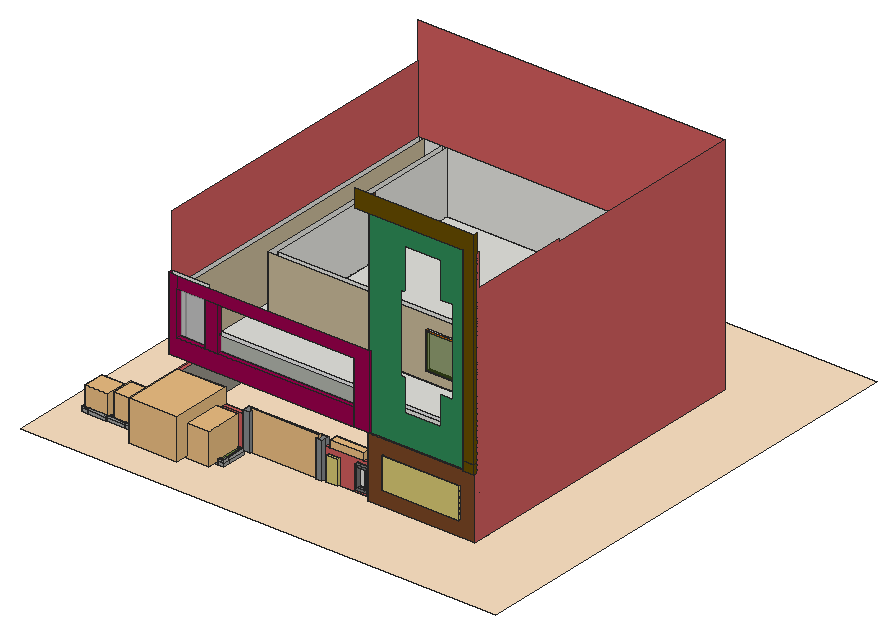
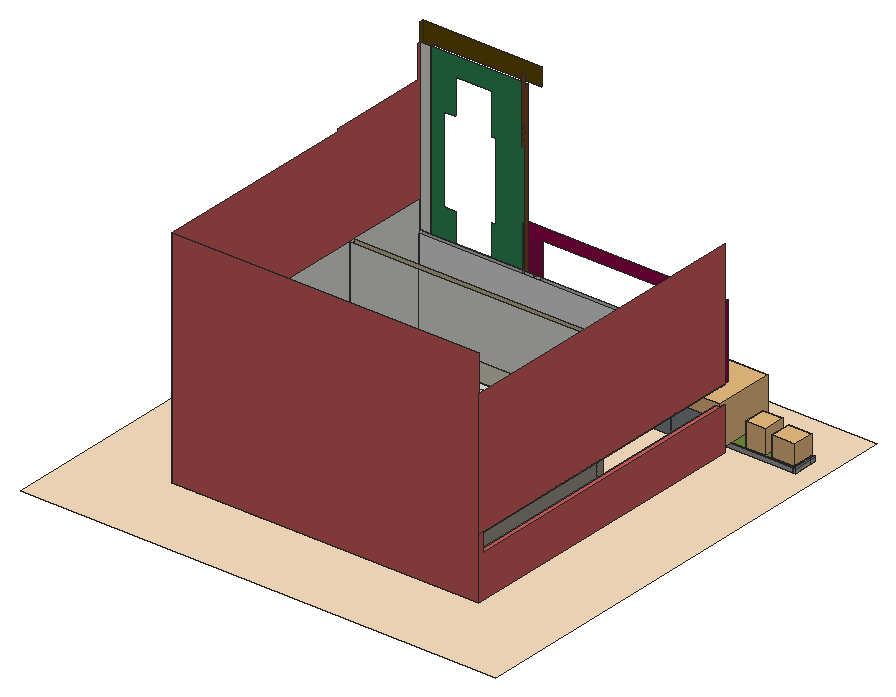
# SketchUp Ruby script. Lengths in inches.
U = 1.inch
M = Sketchup.active_model
def pt(a) = Geom::Point3d.new(a.map { |v| v * U })
def face(e, loops, mat)
  f = e.add_face(loops[0].map { |a| pt(a) })
  loops[1..].each { |l| e.add_face(l.map { |a| pt(a) }).erase! }
  f.material = f.back_material = mat if mat
  f
end
# faces: each face lists its corners as indices into pts; further lists are holes
def faces(e, pts, list, mat = nil) = list.each { |f| face(e, (f[0].is_a?(Array) ? f : [f]).map { |l| l.map { |i| pts[i] } }, mat) }
# xy, xz, yz: faces in a plane at the given z, y or x. An outline is a flat list of corners, or four numbers for a rectangle; further outlines are holes
def ring(l) = l.size == 4 ? [[l[0], l[1]], [l[2], l[1]], [l[2], l[3]], [l[0], l[3]]] : l.each_slice(2).to_a
def flat(e, list, mat, &to3) = list.each { |f| face(e, (f[0].is_a?(Array) ? f : [f]).map { |l| ring(l).map { |u, v| to3.(u, v) } }, mat) }
def xy(e, z, list, mat = nil) = flat(e, list, mat) { |x, y| [x, y, z] }
def xz(e, y, list, mat = nil) = flat(e, list, mat) { |x, z| [x, y, z] }
def yz(e, x, list, mat = nil) = flat(e, list, mat) { |y, z| [x, y, z] }
def lines(e, pts, list) = list.each { |a, b| e.add_line(pt(pts[a]), pt(pts[b])) }
# prism: a flat outline (further loops are holes) pulled along v
def prism(e, loops, v, mat = nil)
  f = face(e, loops, mat); d = Geom::Vector3d.new(v.map { |x| x * U })
  f.pushpull(f.normal.samedirection?(d) ? d.length : -d.length)
end
def box(e, o, s, mat = nil) = prism(e, [[o, [o[0] + s[0], o[1], o[2]], [o[0] + s[0], o[1] + s[1], o[2]], [o[0], o[1] + s[1], o[2]]]], [0, 0, s[2]], mat)
def at(x, y, z, deg = 0) = Geom::Transformation.translation(pt([x, y, z])) * Geom::Transformation.rotation(ORIGIN, Z_AXIS, deg.degrees)
def axes(o, x, y, z) = Geom::Transformation.new([*x, 0, *y, 0, *z, 0, *pt(o).to_a, 1])
def part(name) = M.definitions.add(name)
# library, detail: a bought-in or finely detailed component or shape, given as its bounding box
def library(name, o, s) = part(name).tap { |d| box(d.entities, o, s) }
def detail(e, o, s) = box(e.add_group.entities, o, s)
def put(e, d, t, mat = nil) = e.add_instance(d, t).tap { |i| i.material = mat if mat }
def group(e, t, mat = nil) = e.add_group.tap { |g| g.transformation = t; g.material = mat if mat }.entities
root = M.entities
M.materials.add("PDM_Concrete_02N").color = [160, 160, 159]
M.materials.add("PDM_Concrete_02N-1").color = [160, 160, 159]
M.materials.add("PDM_Grass_03").color = [113, 137, 58]
M.materials.add("[0012_Bisque]").color = [255, 228, 196]
M.materials.add("[0017_IndianRed]").color = [205, 92, 92]
M.materials.add("[0074_SeaGreen]").color = [46, 139, 87]
M.materials.add("[Blacktop Old 01]").color = [132, 136, 139]
M.materials.add("[Color A03]").color = [255, 101, 101]
M.materials.add("[Color C06]").color = [204, 102, 0]
M.materials.add("[Color D08]").color = [102, 76, 0]
M.materials.add("[Color L11]").color = [153, 0, 76]
M.materials.add("[Color M05]").color = [114, 114, 114]
M.materials.add("[Formica Graystone]").color = [149, 146, 135]
M.materials.add("[Mirror 02]").color = [229, 229, 229]
M.materials.add("[Quartz Light Brown]").color = [199, 184, 152]
M.materials.add("[Translucent Glass Blue]").color = [100, 149, 237]
M.materials["[Translucent Glass Blue]"].alpha = 0.5
M.materials.add("[Translucent Glass Dark Green]").color = [62, 91, 5]
M.materials["[Translucent Glass Dark Green]"].alpha = 0.5
M.materials.add("[Translucent Resin Crush Gray]").color = [184, 184, 184]
M.materials["[Translucent Resin Crush Gray]"].alpha = 0.8
M.materials.add("[Wood Board Cork]").color = [215, 201, 115]
M.materials.add("[Wood Floor Parquet]").color = [145, 89, 39]
M.materials.add("[Wood Veneer 01]").color = [120, 70, 37]
c1 = library("gate",[-17.08,19.83,-10.33],[162.44,1,145.04])
c2 = part("255x125 HB kerb.skp\#1")
prism(c2.entities,[[[35.98,4.92,10.04],[35.98,1.15,10.04],[35.98,0.9375,9.96],[35.98,0.8125,9.77],[35.98,0,6.1],[35.98,0,0],[35.98,4.92,0]]],[-35.98,0,0])
c3 = part("305x125 HB external kerb.skp")
xy(c3.entities,0,[[0,0,0,4.92,7.09,4.92,7.09,12.01,12.01,12.01,12.01,0]])
xy(c3.entities,10.04,[[0,1.15,10.86,1.15,10.86,12.01,7.09,12.01,7.09,4.92,0,4.92]])
xz(c3.entities,0,[[0,0,12.01,6.1]])
xz(c3.entities,4.92,[[0,0,7.09,10.04]])
xz(c3.entities,12.01,[[7.09,0,7.09,10.04,10.86,10.04,11.07,9.96,11.19,9.77,12.01,6.1,12.01,0]])
yz(c3.entities,0,[[0,0,0,6.1,0.8125,9.77,0.9375,9.96,1.15,10.04,4.92,10.04,4.92,0]])
yz(c3.entities,7.09,[[4.92,0,12.01,10.04]])
yz(c3.entities,12.01,[[0,0,12.01,6.1]])
p = [[0,0.8125,9.77],[0,0,6.1],[12.01,0,6.1],[11.19,0.8125,9.77],[12.01,12.01,6.1],[11.19,12.01,9.77],
  [0,0.9375,9.96],[11.07,0.9375,9.96],[11.07,12.01,9.96],[0,1.15,10.04],[10.86,1.15,10.04],[10.86,12.01,10.04]]
faces(c3.entities,p,[[0,1,2,3],[3,2,4,5],[6,0,3,7],[7,3,5,8],[9,6,7,10],[10,7,8,11]])
c4 = library("Vase_plant.skp",[-29.68,-24.2,-1.65],[45.82,40.28,40.94])
c5 = library("Aralia.skp\#1",[-13.5,-14.26,0],[27.8,28.98,28.64])
c6 = library("bamboo2.skp\#1",[-10.58,-11.09,0],[94.17,118.22,79.29])
c7 = library("Monstera.skp\#1",[-40.08,-33.23,-2.65],[72.39,71.54,61.35])
c8 = part("flowers")
xy(c8.entities,8.27,[[6.7,5.98,275.44,49.6875]],"PDM_Grass_03")
xz(c8.entities,5.98,[[6.7,0,275.44,8.27]])
xz(c8.entities,49.6875,[[6.7,0,6.9375,8.27],[6.9375,0,275.44,8.27],[6.9375,8.27,275.44,10.04]],"PDM_Concrete_02N")
yz(c8.entities,6.7,[[5.98,0,49.6875,8.27]])
yz(c8.entities,275.44,[[5.98,0,49.6875,8.27]])
p = [[2.02,1.3,0],[2.02,40.67,0]]
lines(c8.entities,p,[[0,1]])
put(c8.entities,c2,at(14.42,1.3,0),"PDM_Concrete_02N-1")
put(c8.entities,c3,at(268.36,1.3,0),"PDM_Concrete_02N-1")
put(c8.entities,c3,at(2.02,13.31,0,-90),"PDM_Concrete_02N-1")
put(c8.entities,c2,at(50.8,1.3,0),"PDM_Concrete_02N-1")
put(c8.entities,c2,at(87.18,1.3,0),"PDM_Concrete_02N-1")
put(c8.entities,c2,at(123.55,1.3,0),"PDM_Concrete_02N-1")
put(c8.entities,c2,at(159.77,1.3,0),"PDM_Concrete_02N-1")
put(c8.entities,c2,at(195.99,1.3,0),"PDM_Concrete_02N-1")
put(c8.entities,c2,at(232.21,1.3,0),"PDM_Concrete_02N-1")
put(c8.entities,c2,at(280.36,13.7,0,90),"PDM_Concrete_02N-1")
put(c8.entities,c2,at(2.02,49.6875,0,-90),"PDM_Concrete_02N-1")
put(c8.entities,c4,at(36.73,27.57,8.27))
put(c8.entities,c5,axes([82.45,23.77,8.27],[1.4,0,0],[0,1.43,0],[0,0,1.63]))
put(c8.entities,c6,at(140.88,-31.91,8.22))
put(c8.entities,c7,at(227.05,18.7,8.27,-180))
c9 = library("APU-ABUS-AZ18C-4-510B-36-CU",[3.59,-10.3125,0.03],[37.07,9.01,7.97])
xy(root,0,[[554.6,156.04,755.73,165.04],[755.73,156.04,765.04,165.04],[308.48,159.04,322.39,165.04],[450.54,159.04,462.67,165.04],[165.04,165.04,165.04,765.04,755.73,765.04,755.73,756.04,174.04,756.04,174.04,174.04,322.39,174.04,322.39,165.04],
  [450.54,165.04,755.73,174.04],[755.73,165.04,755.73,174.04,756.04,174.04,756.04,756.04,755.73,756.04,755.73,765.04,765.04,765.04,765.04,165.04],[755.73,174.04,756.04,241.48],[621.625,241.48,621.625,394.8,631.5,394.8,631.5,249.29,755.73,249.29,755.73,241.48],[755.73,241.48,756.04,249.29],
  [631.5,249.29,755.73,394.8],[755.73,249.29,756.04,394.8],[618.625,309.06,621.625,345.06],[246.86,388.8,252.46,391.8],[484.32,388.8,490.37,391.8],
  [240.41,391.8,276.41,394.8],[477.78,391.8,513.78,394.8],[219.49,394.8,755.73,409.12],[755.73,394.8,756.04,409.12],[219.49,409.12,229.13,756.04],
  [229.13,409.12,755.73,756.04],[755.73,409.12,756.04,756.04]])
xy(root,0,[[[0,0,930.08,930.08],[554.6,156.04,554.6,165.04,462.67,165.04,462.67,159.04,450.54,159.04,450.54,174.04,755.73,174.04,755.73,241.48,621.625,241.48,621.625,309.06,618.625,309.06,618.625,345.06,621.625,345.06,621.625,394.8,513.78,394.8,513.78,391.8,490.37,391.8,490.37,388.8,484.32,388.8,484.32,391.8,477.78,391.8,477.78,394.8,276.41,394.8,276.41,391.8,252.46,391.8,252.46,388.8,246.86,388.8,246.86,391.8,240.41,391.8,240.41,394.8,219.49,394.8,219.49,756.04,174.04,756.04,174.04,174.04,322.39,174.04,322.39,159.04,308.48,159.04,308.48,165.04,165.04,165.04,165.04,765.04,765.04,765.04,765.04,156.04]]],"[0012_Bisque]")
xy(root,2.11,[[471.07,159.04,493.45,165.04]])
xy(root,5.07,[[221.03,159.04,249.4,165.04]])
xy(root,8.16,[[527.11,159.04,550.73,165.04]])
xy(root,12.76,[[531.71,159.04,546.13,165.04]],"[Color M05]")
xy(root,28.7,[[303.38,391.8,330.13,394.8]])
xy(root,29.71,[[584.3,156.04,735.33,159.04]])
xy(root,29.71,[[584.3,153.04,735.33,156.04]],"[Wood Board Cork]")
xy(root,31.87,[[306.55,391.8,326.97,394.8]],"[Color A03]")
xy(root,43.8125,[[557.47,391.8,586.84,394.8]],"[Color A03]")
xy(root,44.95,[[495.58,388.8,502.45,391.8]])
xy(root,48.67,[[471.07,159.04,493.45,165.04]],"[Wood Board Cork]")
xy(root,48.8125,[[531.71,159.04,546.13,165.04]])
xy(root,49.34,[[563,391.8,581.32,394.8]],"[Color A03]")
xy(root,50.98,[[221.03,159.04,249.4,165.04]],"[Wood Board Cork]")
xy(root,53.41,[[527.11,159.04,550.73,165.04]],"[Color M05]")
xy(root,56.85,[[495.58,388.8,502.45,391.8]],"[Wood Veneer 01]")
xy(root,59.5625,[[174.04,165.04,308.48,174.04],[462.67,165.04,554.6,165.04,560.87,174.04,464.34,174.04]],"[0017_IndianRed]")
xy(root,71.5625,[[308.48,159.04,322.39,174.04],[450.54,159.04,462.67,159.04,462.67,165.04,464.34,174.04,450.54,174.04]],"[Blacktop Old 01]")
xy(root,84,[[554.6,165.04,755.73,165.04,755.73,174.04,560.87,174.04],[755.73,174.04,756.04,174.04,756.04,241.48,765.04,243.72,755.73,243.72]])
xy(root,84,[[165.04,165.04,174.04,756.04]],"[0017_IndianRed]")
xy(root,84,[[618.625,309.06,621.625,345.06]],"[Wood Floor Parquet]")
xy(root,84,[[246.86,388.8,252.46,391.8],[484.32,388.8,490.37,391.8],[240.41,391.8,276.41,394.8],[477.78,391.8,513.78,394.8]],"[Wood Veneer 01]")
xy(root,85.8125,[[563,391.8,581.32,394.8]])
xy(root,87.35,[[306.55,391.8,326.97,394.8]])
xy(root,89.48,[[584.3,156.04,735.33,159.04]])
xy(root,89.48,[[584.3,153.04,735.33,156.04]],"[Wood Board Cork]")
xy(root,90.52,[[303.38,391.8,330.13,394.8]],"[Color A03]")
xy(root,91.34,[[557.47,391.8,586.84,394.8]],"[Color A03]")
xy(root,119.1875,[[743.6,153.04,765.04,156.04],[743.6,156.04,765.04,159.04],[165.04,165.04,756.04,174.04],[174.04,174.04,174.04,756.04,219.49,756.04,219.49,331.59,430.45,331.59,430.45,328.59,441.07,328.59,441.07,324.28,448.45,324.28,448.45,328.59,466.45,328.59,466.45,331.59,621.625,331.59,621.625,241.48,756.04,241.48,756.04,174.04]])
xy(root,119.1875,[[165.04,174.04,174.04,756.04]],"[0017_IndianRed]")
xy(root,119.1875,[[554.6,156.04,743.6,159.04]],"[Wood Veneer 01]")
xy(root,119.4375,[[165.04,165.04,756.04,174.04]])
xy(root,119.875,[[523.3,165.04,534.36,169.69,536.32,165.04]])
xy(root,119.875,[[181.38,156.04,181.38,165.04,523.3,165.04,527.08,156.04],[527.08,156.04,523.3,165.04,527.13,165.04,527.13,156.04],[527.13,156.04,559.05,165.04]],"[Color L11]")
xy(root,120,[[174.04,165.23,755.73,174.04],[755.73,165.23,756.04,174.04],[174.04,174.04,185.29,756.04],[755.73,174.04,756.04,241.48],[621.625,241.48,755.73,241.48,755.73,243.72,756.04,243.72,756.04,249.29,631.5,249.29,631.5,331.59,621.625,331.59],
  [755.73,241.48,756.04,243.72],[756.04,241.48,756.04,243.72,765.04,243.72],[631.5,249.29,756.04,331.59],[441.07,324.28,448.45,324.28,448.45,328.59,466.45,328.59,466.45,331.59,430.45,331.59,430.45,328.59,441.07,328.59],[219.9375,331.59,621.625,342.77],
  [621.625,331.59,631.5,342.77],[631.5,331.59,756.04,342.77],[621.625,342.77,631.5,394.8],[631.5,342.77,756.04,394.8],[219.49,394.8,229.13,409.12],
  [229.13,394.8,756.04,409.12],[219.49,409.12,229.13,756.04],[229.13,409.12,756.04,756.04]])
xy(root,120,[[165.04,156.04,181.38,165.04]],"[Color L11]")
xy(root,120,[[219.49,331.59,219.49,394.8,229.13,394.8,229.13,342.77,219.9375,342.77,219.9375,331.59],[229.13,342.77,621.625,394.8]],"[Formica Graystone]")
xy(root,121,[[165.04,174.04,174.04,756.04]])
xy(root,122.25,[[174.04,174.04,756.04,174.04,756.04,241.48,621.625,241.48,621.625,331.59,466.45,331.59,466.45,328.59,448.45,328.59,448.45,324.28,441.07,324.28,441.07,328.59,430.45,328.59,430.45,331.59,219.49,331.59,219.49,756.04,174.04,756.04]])
xy(root,137.6875,[[743.6,153.04,765.04,159.04]])
xy(root,142.4,[[530.78,328.59,675.97,331.59]])
xy(root,145.4,[[533.78,326.59,672.97,328.59],[533.78,328.59,672.97,331.59]])
xy(root,154.27,[[236.6,156.04,260.92,165.04]])
xy(root,154.27,[[181.38,156.04,236.6,165.04],[260.92,156.04,527.13,165.04]],"[Color L11]")
xz(root,153.04,[[743.6,119.1875,765.04,137.6875],[743.6,137.6875,765.04,137.6875,765.04,541.25,531.67,541.25,531.67,506.1875,743.6,506.1875]],"[Color D08]")
xz(root,153.04,[[584.3,29.71,735.33,89.48]],"[Wood Board Cork]")
xz(root,156.04,[[527.08,119.875,527.13,154.27]])
xz(root,156.04,[[181.38,119.875,527.08,119.875,527.08,154.27,181.38,154.27,181.38,262.875,165.04,262.875,165.04,120,181.38,120],[527.13,119.875,559.05,119.875,559.05,262.875,181.38,262.875,181.38,240,527.08,240,527.08,154.27,527.13,154.27],[236.6,154.27,260.92,240]],"[Color L11]")
xz(root,156.04,[[[554.6,0,765.04,119.1875],[584.3,29.71,735.33,89.48]]],"[Wood Veneer 01]")
xz(root,159.04,[[584.3,29.71,735.33,89.48],[743.6,119.1875,765.04,137.6875],[743.6,137.6875,765.04,506.1875]])
xz(root,159.04,[[[554.6,119.1875,743.6,506.1875],[623.84,177.05,623.84,237.91,616.375,237.91,616.375,389.91,623.84,389.91,623.84,469.24,695.78,469.24,695.78,400.38,718.71,400.38,718.71,232.57,695.78,232.57,695.78,177.05]]],"[0074_SeaGreen]")
xz(root,159.04,[[308.48,0,322.39,71.5625],[450.54,0,462.67,71.5625]],"[Blacktop Old 01]")
xz(root,159.04,[[[527.11,8.16,550.73,53.41],[531.71,12.76,546.13,48.8125]]],"[Color M05]")
xz(root,159.04,[[471.07,2.11,493.45,48.67],[221.03,5.07,249.4,50.98]],"[Wood Board Cork]")
xz(root,165.04,[[554.6,0,755.73,84],[471.07,2.11,493.45,48.67],[221.03,5.07,249.4,50.98],[[527.11,8.16,550.73,53.41],[531.71,12.76,546.13,48.8125]],[531.71,12.76,546.13,48.8125],
  [554.6,84,755.73,119.1875],[165.04,119.1875,554.6,119.4375],[554.6,119.1875,755.73,119.4375],[755.73,119.1875,756.04,119.4375],[756.04,119.1875,765.04,119.4375],
  [554.6,119.4375,554.6,119.875,559.05,119.875,559.05,120,755.73,120,755.73,119.4375],[755.73,119.4375,765.04,120],[181.38,119.875,523.3,119.875,523.3,154.27,260.92,154.27,260.92,153.875,236.6,153.875,236.6,154.27,181.38,154.27],[523.3,119.875,527.13,154.27],[527.13,119.875,554.6,120],
  [554.6,119.875,559.05,120],[165.04,120,165.04,262.875,236.6,262.875,236.6,240,174.04,240,174.04,120],[174.04,120,181.38,181.3125],[527.13,120,554.6,120,554.6,181.3125,523.3,181.3125,523.3,154.27,527.13,154.27],[554.6,120,559.05,181.3125],
  [554.6,120,559.05,262.875],[559.05,120,755.73,181.3125],[236.6,153.875,260.92,154.27],[236.6,154.27,260.92,155.125],[236.6,155.125,260.92,172.75],
  [236.6,172.75,260.92,181.3125]])
xz(root,165.04,[[[165.04,0,308.48,0,308.48,59.5625,174.04,59.5625,174.04,84,165.04,84],[221.03,5.07,249.4,50.98]],[[462.67,0,554.6,59.5625],[527.11,8.16,550.73,53.41],[471.07,2.11,493.45,48.67]]],"[0017_IndianRed]")
xz(root,165.04,[[260.92,154.27,523.3,181.3125]],"[Translucent Glass Dark Green]")
xz(root,165.23,[[174.04,120,756.04,120,756.04,181.3125,236.6875,181.3125,236.6875,240,174.04,240]],"[Translucent Resin Crush Gray]")
xz(root,174.04,[[165.04,119.1875,174.04,119.4375],[174.04,119.1875,756.04,119.4375],[165.04,119.4375,174.04,121],[174.04,119.4375,756.04,120],[174.04,120,185.29,122.25],
  [185.29,120,756.04,122.25],[174.04,122.25,185.29,240]])
xz(root,174.04,[[174.04,0,322.39,59.5625],[450.54,0,450.54,71.5625,464.34,71.5625,464.34,59.5625,560.87,59.5625,560.87,84,756.04,84,756.04,0],[308.48,59.5625,322.39,71.5625]],"[Blacktop Old 01]")
xz(root,174.04,[[185.29,122.25,185.29,240,241.08,240,241.08,182.0625,756.04,182.0625,756.04,122.25]],"[Mirror 02]")
xz(root,241.48,[[621.625,119.1875,756.04,120],[621.625,120,756.04,122.25]])
xz(root,241.48,[[621.625,0,756.04,119.1875]],"[Formica Graystone]")
xz(root,249.29,[[631.5,0,756.04,120]])
xz(root,309.06,[[618.625,0,621.625,84]],"[Wood Floor Parquet]")
xz(root,324.28,[[441.07,119.1875,448.45,120],[441.07,120,448.45,122.25]])
xz(root,324.28,[[441.07,122.25,448.45,204],[434.68,161.93,435.69,161.99,436.64,162.32,437.48,162.88,438.15,163.64,438.6,164.55,438.8,165.54,438.73,166.55,438.41,167.51,437.84,168.35,437.08,169.02,436.18,169.46,435.19,169.66,434.18,169.6,433.22,169.27,432.375,168.71,431.71,167.95,431.26,167.04,431.0625,166.05,431.13,165.04,431.45,164.08,432.02,163.24,432.78,162.57,433.68,162.125]],"[Wood Floor Parquet]")
xz(root,326.59,[[533.78,145.4,672.97,212.33]],"[Translucent Glass Dark Green]")
xz(root,328.59,[[430.45,119.1875,441.07,120],[448.45,119.1875,466.45,120],[430.45,120,441.07,122.25],[448.45,120,466.45,122.25]])
xz(root,328.59,[[[530.78,142.4,675.97,215.33],[533.78,145.4,672.97,212.33]]],"[Color C06]")
xz(root,328.59,[[[430.45,122.25,441.07,204],[434.68,161.93,433.68,162.125,432.78,162.57,432.02,163.24,431.45,164.08,431.13,165.04,431.0625,166.05,431.26,167.04,431.71,167.95,432.375,168.71,433.22,169.27,434.18,169.6,435.19,169.66,436.18,169.46,437.08,169.02,437.84,168.35,438.41,167.51,438.73,166.55,438.8,165.54,438.6,164.55,438.15,163.64,437.48,162.88,436.64,162.32,435.69,161.99]],[448.45,122.25,466.45,204]],"[Wood Floor Parquet]")
xz(root,331.59,[[219.49,119.1875,219.9375,120],[219.9375,119.1875,430.45,120],[466.45,119.1875,621.625,120],[219.49,120,219.9375,122.25],[219.9375,120,430.45,122.25],
  [430.45,120,466.45,204],[466.45,120,621.625,122.25],[[530.78,142.4,675.97,215.33],[533.78,145.4,672.97,212.33]]])
xz(root,331.59,[[[621.625,120,756.04,120,756.04,240,219.49,240,219.49,122.25,430.45,122.25,430.45,204,466.45,204,466.45,122.25,621.625,122.25],[530.78,142.4,675.97,215.33]]],"[Quartz Light Brown]")
xz(root,342.77,[[229.13,120,621.625,240],[621.625,120,756.04,240]])
xz(root,345.06,[[618.625,0,621.625,84]],"[Wood Floor Parquet]")
xz(root,388.8,[[246.86,0,252.46,84],[484.32,0,490.37,84],[263.52,43.59,269.85,47.24,269.85,54.56,263.52,58.21,257.18,54.56,257.18,47.24],[495.58,44.95,502.45,44.95,505.89,50.9,502.45,56.85,495.58,56.85,492.14,50.9]],"[Wood Veneer 01]")
xz(root,391.8,[[246.86,0,252.46,84],[484.32,0,490.37,84],[263.52,43.59,257.18,47.24,257.18,54.56,263.52,58.21,269.85,54.56,269.85,47.24],[495.58,44.95,492.14,50.9,495.58,56.85,502.45,56.85,505.89,50.9,502.45,44.95]])
xz(root,391.8,[[[303.38,28.7,330.13,90.52],[306.55,31.87,326.97,87.35]],[[557.47,43.8125,586.84,91.34],[563,49.34,581.32,85.8125]]],"[Color A03]")
xz(root,391.8,[[240.41,0,246.86,84],[[252.46,0,276.41,84],[263.52,43.59,257.18,47.24,257.18,54.56,263.52,58.21,269.85,54.56,269.85,47.24]],[477.78,0,484.32,84],[[490.37,0,513.78,84],[495.58,44.95,492.14,50.9,495.58,56.85,502.45,56.85,505.89,50.9,502.45,44.95]]],"[Wood Veneer 01]")
xz(root,394.8,[[240.41,0,276.41,84],[477.78,0,513.78,84],[621.625,0,631.5,120],[631.5,0,756.04,120],[[303.38,28.7,330.13,90.52],[306.55,31.87,326.97,87.35]],
  [[557.47,43.8125,586.84,91.34],[563,49.34,581.32,85.8125]]])
xz(root,394.8,[[[219.49,0,240.41,0,240.41,84,276.41,84,276.41,0,477.78,0,477.78,84,513.78,84,513.78,0,621.625,0,621.625,120,219.49,120],[303.38,28.7,330.13,90.52],[557.47,43.8125,586.84,91.34]]],"[Formica Graystone]")
xz(root,394.8,[[306.55,31.87,326.97,87.35],[563,49.34,581.32,85.8125]],"[Translucent Glass Blue]")
xz(root,409.12,[[219.49,0,229.13,120],[229.13,0,756.04,120]])
xz(root,756.04,[[219.49,0,229.13,120],[229.13,0,756.04,120],[165.04,119.1875,174.04,120],[174.04,119.1875,219.49,120],[165.04,120,174.04,121],
  [174.04,120,185.29,122.25],[185.29,120,219.49,122.25],[219.49,120,229.13,240],[229.13,120,756.04,240],[174.04,122.25,185.29,240],
  [185.29,122.25,219.49,240]])
xz(root,756.04,[[174.04,0,219.49,107.75],[165.04,84,174.04,107.75],[165.04,107.75,219.49,119.1875]],"[0017_IndianRed]")
xz(root,765.04,[[165.04,0,765.04,437.75]],"[0017_IndianRed]")
yz(root,165.04,[[165.04,119.1875,174.04,119.4375]])
yz(root,165.04,[[165.04,0,165.04,84,756.04,84,756.04,120,765.04,120,765.04,0],[174.04,119.1875,756.04,120],[165.04,120,165.04,365.75,765.04,365.75,765.04,120,756.04,120,756.04,121,174.04,121,174.04,120],[174.04,120,756.04,121]],"[0017_IndianRed]")
yz(root,165.04,[[156.04,120,165.04,262.875]],"[Color L11]")
yz(root,174.04,[[174.04,119.1875,756.04,120],[165.23,120,174.04,240],[174.04,120,756.04,121],[174.04,121,756.04,122.25],[174.04,122.25,756.04,240]])
yz(root,174.04,[[174.04,0,756.04,0,756.04,84,165.04,84,165.04,59.5625,174.04,59.5625]],"[Formica Graystone]")
yz(root,181.38,[[156.04,119.875,165.04,120]])
yz(root,181.38,[[156.04,154.27,165.04,240]],"[Color L11]")
yz(root,185.29,[[174.04,120,756.04,240]],"[Quartz Light Brown]")
yz(root,219.49,[[331.59,119.1875,394.8,120],[394.8,119.1875,409.12,120],[409.12,119.1875,756.04,120],[331.59,120,394.8,122.25],[394.8,120,409.12,122.25],
  [409.12,120,756.04,122.25],[331.59,122.25,756.04,240]])
yz(root,219.49,[[394.8,0,409.12,107.75],[409.12,0,756.04,107.75],[394.8,107.75,409.12,116.25],[409.12,107.75,756.04,119.1875],[394.8,116.25,409.12,119.1875]],"[Formica Graystone]")
yz(root,221.03,[[159.04,5.07,165.04,50.98]],"[Wood Board Cork]")
yz(root,229.13,[[409.12,0,756.04,120],[342.77,120,756.04,240]])
yz(root,236.6,[[156.04,154.27,165.04,155.125]])
yz(root,236.6,[[156.04,155.125,165.04,240]],"[Color L11]")
yz(root,240.41,[[391.8,0,394.8,84]],"[Wood Veneer 01]")
yz(root,246.86,[[388.8,0,391.8,84]],"[Wood Veneer 01]")
yz(root,249.4,[[159.04,5.07,165.04,50.98]],"[Wood Board Cork]")
yz(root,252.46,[[388.8,0,391.8,84]],"[Wood Veneer 01]")
yz(root,257.18,[[388.8,47.24,391.8,54.56]],"[Wood Veneer 01]")
yz(root,260.92,[[[156.04,154.27,165.04,240],[161.8,182.97,161,183.08,160.24,183.39,159.6,183.89,159.1,184.54,158.79,185.29,158.68,186.1,158.79,186.91,159.1,187.66,159.6,188.31,160.24,188.8,161,189.12,161.8,189.22,162.61,189.12,163.37,188.8,164.01,188.31,164.51,187.66,164.82,186.91,164.93,186.1,164.82,185.29,164.51,184.54,164.01,183.89,163.37,183.39,162.61,183.08]]],"[Color L11]")
yz(root,269.85,[[388.8,47.24,391.8,54.56]],"[Wood Veneer 01]")
yz(root,276.41,[[391.8,0,394.8,84]],"[Wood Veneer 01]")
yz(root,303.38,[[391.8,28.7,394.8,90.52]],"[Color A03]")
yz(root,306.55,[[391.8,31.87,394.8,87.35]],"[Color A03]")
yz(root,308.48,[[159.04,0,159.04,71.5625,174.04,71.5625,174.04,59.5625,165.04,59.5625,165.04,0]],"[Blacktop Old 01]")
yz(root,322.39,[[159.04,0,174.04,71.5625]],"[Blacktop Old 01]")
yz(root,326.97,[[391.8,31.87,394.8,87.35]],"[Color A03]")
yz(root,330.13,[[391.8,28.7,394.8,90.52]],"[Color A03]")
yz(root,430.45,[[328.59,119.1875,331.59,120],[328.59,120,331.59,122.25]])
yz(root,430.45,[[328.59,122.25,331.59,204]],"[Wood Floor Parquet]")
yz(root,441.07,[[324.28,119.1875,328.59,120],[324.28,120,328.59,122.25]])
yz(root,441.07,[[324.28,122.25,328.59,204]],"[Wood Floor Parquet]")
yz(root,448.45,[[324.28,119.1875,328.59,120],[324.28,120,328.59,122.25]])
yz(root,448.45,[[324.28,122.25,328.59,204]],"[Wood Floor Parquet]")
yz(root,450.54,[[159.04,0,174.04,71.5625]],"[Blacktop Old 01]")
yz(root,462.67,[[159.04,0,165.04,71.5625]],"[Blacktop Old 01]")
yz(root,466.45,[[328.59,119.1875,331.59,120],[328.59,120,331.59,122.25]])
yz(root,466.45,[[328.59,122.25,331.59,204]],"[Wood Floor Parquet]")
yz(root,471.07,[[159.04,2.11,165.04,48.67]],"[Wood Board Cork]")
yz(root,477.78,[[391.8,0,394.8,84]],"[Wood Veneer 01]")
yz(root,484.32,[[388.8,0,391.8,84]],"[Wood Veneer 01]")
yz(root,490.37,[[388.8,0,391.8,84]],"[Wood Veneer 01]")
yz(root,493.45,[[159.04,2.11,165.04,48.67]],"[Wood Board Cork]")
yz(root,513.78,[[391.8,0,394.8,84]],"[Wood Veneer 01]")
yz(root,527.11,[[159.04,8.16,165.04,53.41]],"[Color M05]")
yz(root,527.13,[[156.04,119.875,165.04,154.27]])
yz(root,530.78,[[328.59,142.4,331.59,215.33]],"[Color C06]")
yz(root,531.71,[[159.04,12.76,165.04,48.8125]],"[Color M05]")
yz(root,533.78,[[328.59,145.4,331.59,212.33]])
yz(root,533.78,[[326.59,145.4,328.59,212.33]],"[Color C06]")
yz(root,546.13,[[159.04,12.76,165.04,48.8125]],"[Color M05]")
yz(root,550.73,[[159.04,8.16,165.04,53.41]],"[Color M05]")
yz(root,554.6,[[[156.04,0,156.04,119.1875,159.04,119.1875,159.04,506.1875,165.04,506.1875,165.04,531,174.04,531,174.04,401.875,165.04,401.875,165.04,0],[170.29,407.24,171.23,407.36,172.11,407.73,172.86,408.3,173.43,409.05,173.79,409.93,173.92,410.87,173.79,411.8,173.43,412.68,172.86,413.43,172.11,414.01,171.23,414.37,170.29,414.49,169.35,414.37,168.48,414.01,167.73,413.43,167.15,412.68,166.79,411.8,166.67,410.87,166.79,409.93,167.15,409.05,167.73,408.3,168.48,407.73,169.35,407.36],[170.29,420.3,171.23,420.43,172.11,420.79,172.86,421.37,173.43,422.12,173.79,422.99,173.92,423.93,173.79,424.87,173.43,425.74,172.86,426.49,172.11,427.07,171.23,427.43,170.29,427.55,169.35,427.43,168.48,427.07,167.73,426.49,167.15,425.74,166.79,424.87,166.67,423.93,166.79,422.99,167.15,422.12,167.73,421.37,168.48,420.79,169.35,420.43],[170.29,430.24,171.23,430.36,172.11,430.73,172.86,431.3,173.43,432.05,173.79,432.93,173.92,433.87,173.79,434.8,173.43,435.68,172.86,436.43,172.11,437.01,171.23,437.37,170.29,437.49,169.35,437.37,168.48,437.01,167.73,436.43,167.15,435.68,166.79,434.8,166.67,433.87,166.79,432.93,167.15,432.05,167.73,431.3,168.48,430.73,169.35,430.36]]],"[Wood Veneer 01]")
yz(root,557.47,[[391.8,43.8125,394.8,91.34]],"[Color A03]")
yz(root,559.05,[[156.04,119.875,165.04,262.875]],"[Color L11]")
yz(root,563,[[391.8,49.34,394.8,85.8125]],"[Color A03]")
yz(root,581.32,[[391.8,49.34,394.8,85.8125]],"[Color A03]")
yz(root,584.3,[[156.04,29.71,159.04,89.48]])
yz(root,584.3,[[153.04,29.71,156.04,89.48]],"[Wood Board Cork]")
yz(root,586.84,[[391.8,43.8125,394.8,91.34]],"[Color A03]")
yz(root,615.625,[[338.11,45.41,336.62,45.61,335.23,46.18,334.04,47.1,333.125,48.29,332.55,49.67,332.36,51.16,332.55,52.65,333.125,54.04,334.04,55.23,335.23,56.14,336.62,56.72,338.11,56.91,339.59,56.72,340.98,56.14,342.17,55.23,343.09,54.04,343.66,52.65,343.86,51.16,343.66,49.67,343.09,48.29,342.17,47.1,340.98,46.18,339.59,45.61]],"[Wood Floor Parquet]")
yz(root,618.625,[[338.11,45.41,339.59,45.61,340.98,46.18,342.17,47.1,343.09,48.29,343.66,49.67,343.86,51.16,343.66,52.65,343.09,54.04,342.17,55.23,340.98,56.14,339.59,56.72,338.11,56.91,336.62,56.72,335.23,56.14,334.04,55.23,333.125,54.04,332.55,52.65,332.36,51.16,332.55,49.67,333.125,48.29,334.04,47.1,335.23,46.18,336.62,45.61]])
yz(root,618.625,[[[309.06,0,345.06,84],[338.11,45.41,339.59,45.61,340.98,46.18,342.17,47.1,343.09,48.29,343.66,49.67,343.86,51.16,343.66,52.65,343.09,54.04,342.17,55.23,340.98,56.14,339.59,56.72,338.11,56.91,336.62,56.72,335.23,56.14,334.04,55.23,333.125,54.04,332.55,52.65,332.36,51.16,332.55,49.67,333.125,48.29,334.04,47.1,335.23,46.18,336.62,45.61]]],"[Wood Floor Parquet]")
yz(root,621.625,[[309.06,0,345.06,84],[241.48,119.1875,331.59,120],[241.48,120,331.59,122.25]])
yz(root,621.625,[[241.48,0,241.48,119.1875,331.59,119.1875,331.59,120,394.8,120,394.8,0,345.06,0,345.06,84,309.06,84,309.06,0]],"[Formica Graystone]")
yz(root,631.5,[[249.29,0,394.8,120]])
yz(root,672.97,[[326.59,145.4,328.59,212.33],[328.59,145.4,331.59,212.33]])
yz(root,675.97,[[328.59,142.4,331.59,215.33]])
yz(root,735.33,[[156.04,29.71,159.04,89.48]])
yz(root,735.33,[[153.04,29.71,156.04,89.48]],"[Wood Board Cork]")
yz(root,743.6,[[153.04,119.1875,159.04,137.6875],[153.04,137.6875,159.04,506.1875]],"[Color D08]")
yz(root,756.04,[[174.04,0,241.48,84],[241.48,0,249.29,120],[249.29,0,394.8,120],[394.8,0,409.12,120],[409.12,0,756.04,120],
  [165.04,119.1875,174.04,119.4375],[174.04,119.1875,241.48,120],[165.23,120,174.04,182.0625],[174.04,120,241.48,122.25],[241.48,120,241.48,122.25,174.04,122.25,174.04,240,331.59,240,331.59,120],
  [331.59,120,342.77,240],[342.77,120,756.04,240]])
yz(root,765.04,[[156.04,0,765.04,0,765.04,437.75,360.73,437.75,360.73,442.375,165.04,442.375,165.04,506.1875,159.04,506.1875,159.04,119.1875,156.04,119.1875]],"[0017_IndianRed]")
yz(root,765.04,[[153.04,119.1875,159.04,137.6875],[153.04,137.6875,159.04,541.25]],"[Color D08]")
p = [[257.18,391.8,47.24],[263.52,391.8,43.59],[263.52,388.8,43.59],[257.18,388.8,47.24],[269.85,391.8,47.24],[269.85,388.8,47.24],
  [492.14,391.8,50.9],[495.58,391.8,44.95],[495.58,388.8,44.95],[492.14,388.8,50.9],[502.45,391.8,44.95],[505.89,391.8,50.9],
  [505.89,388.8,50.9],[502.45,388.8,44.95],[618.625,338.11,45.41],[618.625,336.62,45.61],[615.625,336.62,45.61],[615.625,338.11,45.41],
  [618.625,339.59,45.61],[615.625,339.59,45.61],[618.625,335.23,46.18],[615.625,335.23,46.18],[618.625,340.98,46.18],[615.625,340.98,46.18],
  [618.625,334.04,47.1],[615.625,334.04,47.1],[618.625,342.17,47.1],[615.625,342.17,47.1],[618.625,333.125,48.29],[615.625,333.125,48.29],
  [618.625,343.09,48.29],[615.625,343.09,48.29],[618.625,332.55,49.67],[615.625,332.55,49.67],[618.625,343.66,49.67],[615.625,343.66,49.67],
  [618.625,332.36,51.16],[615.625,332.36,51.16],[618.625,343.86,51.16],[615.625,343.86,51.16],[495.58,391.8,56.85],[495.58,388.8,56.85],
  [502.45,391.8,56.85],[502.45,388.8,56.85],[618.625,332.55,52.65],[615.625,332.55,52.65],[618.625,343.66,52.65],[615.625,343.66,52.65],
  [618.625,333.125,54.04],[615.625,333.125,54.04],[618.625,343.09,54.04],[615.625,343.09,54.04],[618.625,334.04,55.23],[615.625,334.04,55.23],
  [618.625,342.17,55.23],[615.625,342.17,55.23],[263.52,391.8,58.21],[257.18,391.8,54.56],[257.18,388.8,54.56],[263.52,388.8,58.21],
  [269.85,391.8,54.56],[269.85,388.8,54.56],[618.625,335.23,56.14],[615.625,335.23,56.14],[618.625,340.98,56.14],[615.625,340.98,56.14],
  [618.625,336.62,56.72],[615.625,336.62,56.72],[618.625,339.59,56.72],[615.625,339.59,56.72],[618.625,338.11,56.91],[615.625,338.11,56.91],
  [462.67,165.04,59.5625],[464.34,174.04,59.5625],[464.34,174.04,71.5625],[462.67,165.04,71.5625],[554.6,165.04,84],[560.87,174.04,84],
  [560.87,174.04,59.5625],[554.6,165.04,59.5625],[527.08,156.04,240],[523.3,165.04,240],[523.3,165.04,181.3125],[523.3,165.04,154.27],
  [523.3,165.04,120],[523.3,165.04,119.875],[527.08,156.04,119.875],[527.08,156.04,154.27],[523.75,165.23,120],[534.36,169.69,120],
  [534.36,169.69,119.875],[523.75,165.23,181.3125],[534.36,169.69,181.3125],[433.68,328.59,162.125],[434.68,328.59,161.93],[434.68,324.28,161.93],
  [433.68,324.28,162.125],[435.69,328.59,161.99],[435.69,324.28,161.99],[436.64,328.59,162.32],[436.64,324.28,162.32],[432.78,328.59,162.57],
  [432.78,324.28,162.57],[437.48,328.59,162.88],[437.48,324.28,162.88],[432.02,328.59,163.24],[432.02,324.28,163.24],[438.15,328.59,163.64],
  [438.15,324.28,163.64],[431.45,328.59,164.08],[431.45,324.28,164.08],[438.6,328.59,164.55],[438.6,324.28,164.55],[431.13,328.59,165.04],
  [431.13,324.28,165.04],[438.8,328.59,165.54],[438.8,324.28,165.54],[431.0625,328.59,166.05],[431.0625,324.28,166.05],[438.73,328.59,166.55],
  [438.73,324.28,166.55],[431.26,328.59,167.04],[431.26,324.28,167.04],[438.41,328.59,167.51],[438.41,324.28,167.51],[431.71,328.59,167.95],
  [431.71,324.28,167.95],[437.84,328.59,168.35],[437.84,324.28,168.35],[432.375,328.59,168.71],[432.375,324.28,168.71],[437.08,328.59,169.02],
  [437.08,324.28,169.02],[433.22,328.59,169.27],[433.22,324.28,169.27],[436.18,328.59,169.46],[436.18,324.28,169.46],[434.18,328.59,169.6],
  [434.18,324.28,169.6],[435.19,328.59,169.66],[435.19,324.28,169.66],[466.45,331.59,107.75],[466.45,328.59,107.75],[219.49,331.59,107.75],
  [219.9375,331.59,107.75],[755.73,165.04,120],[755.73,165.23,120],[755.73,243.72,120],[755.73,243.72,84],[538.15,160.69,240],
  [538.15,160.69,119.875],[755.73,165.04,84],[765.04,165.04,84],[260.92,165.04,153.875],[260.92,156.04,153.875],[236.6,165.04,153.875],
  [236.6,156.04,153.875]]
faces(root,p,[[0,1,2,3],[1,4,5,2],[6,7,8,9],[10,11,12,13],[40,6,9,41],[11,42,43,12],[56,57,58,59],[60,56,59,61]],"[Wood Veneer 01]")
faces(root,p,[[14,15,16,17],[18,14,17,19],[15,20,21,16],[22,18,19,23],[20,24,25,21],[26,22,23,27],[24,28,29,25],[30,26,27,31],
  [28,32,33,29],[34,30,31,35],[32,36,37,33],[38,34,35,39],[36,44,45,37],[46,38,39,47],[44,48,49,45],[50,46,47,51],
  [48,52,53,49],[54,50,51,55],[52,62,63,53],[64,54,55,65],[62,66,67,63],[68,64,65,69],[66,70,71,67],[70,68,69,71],
  [93,94,95,96],[94,97,98,95],[97,99,100,98],[101,93,96,102],[99,103,104,100],[105,101,102,106],[103,107,108,104],[109,105,106,110],
  [107,111,112,108],[113,109,110,114],[111,115,116,112],[117,113,114,118],[115,119,120,116],[121,117,118,122],[119,123,124,120],[125,121,122,126],
  [123,127,128,124],[129,125,126,130],[127,131,132,128],[133,129,130,134],[131,135,136,132],[137,133,134,138],[135,139,140,136],[139,137,138,140]],"[Wood Floor Parquet]")
faces(root,p,[[72,73,74,75]],"[Blacktop Old 01]")
faces(root,p,[[76,77,78,79],[85,84,88,89,90],[83,82,91,92,89,88,84]])
faces(root,p,[[80,81,82,83,84,85,86,87]],"[Color L11]")
lines(root,p,[[141,142],[143,144],[145,146],[147,148],[149,150],[151,152],[153,154],[155,156]])
put(root,c1,axes([335.0625,91.95,3.03],[0.819,0,0],[0,3.549,0],[0,0,0.546]))
put(root,c8,at(37.53,98.74,0))
put(root,c9,axes([467.3,183.19,59.51],[1.76,0,0],[0,1.76,0],[0,0,1.76]))
